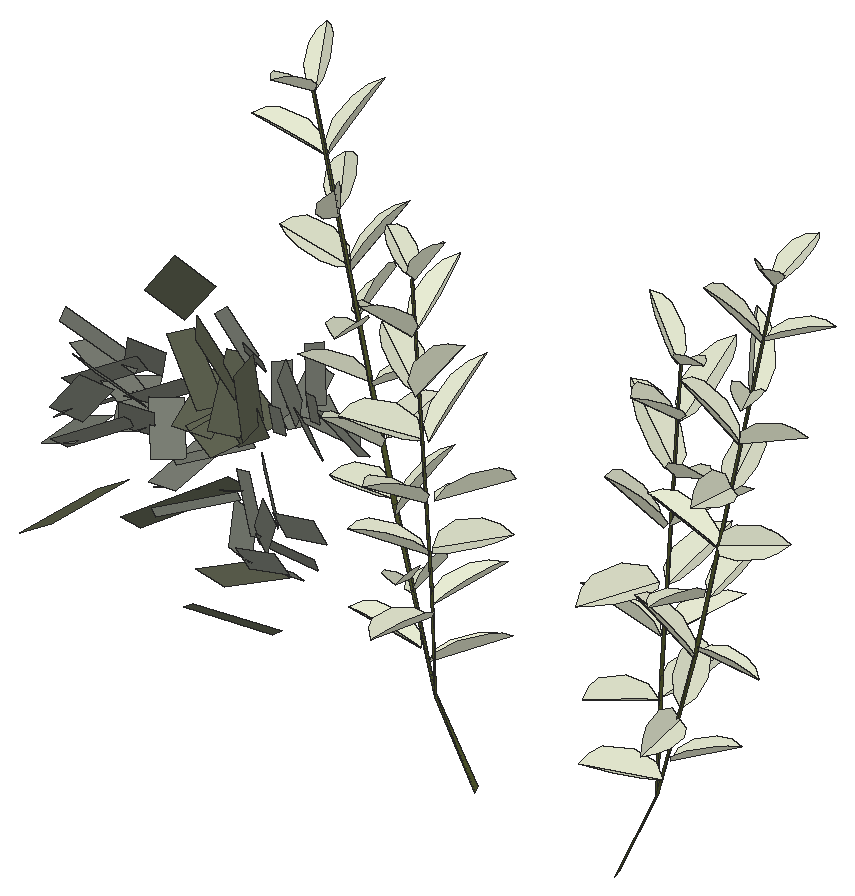
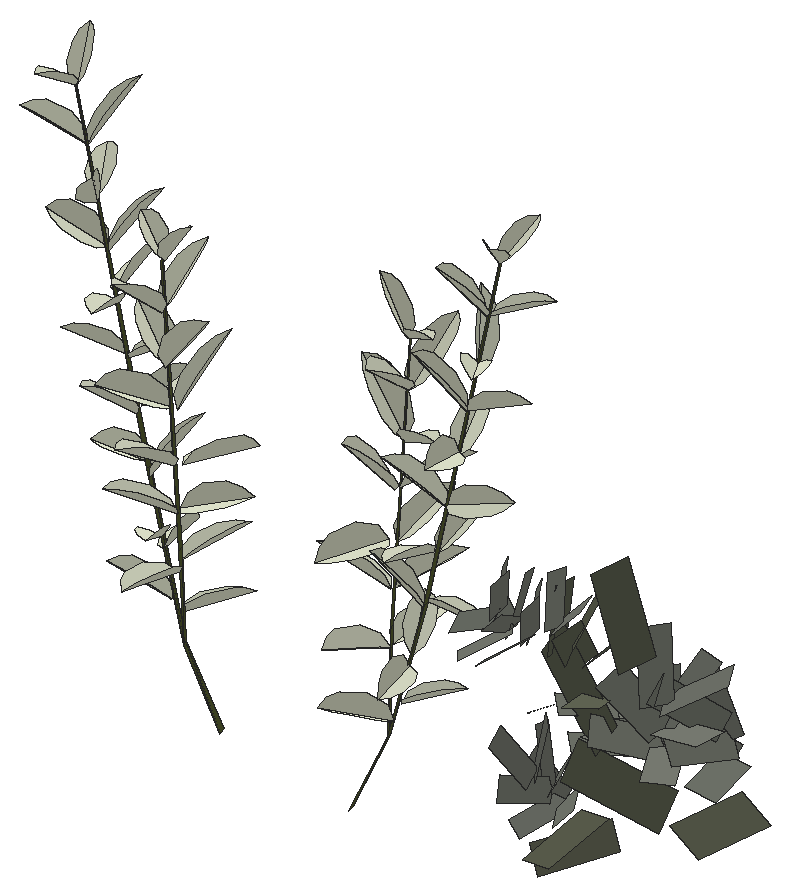
# SketchUp Ruby script. Lengths in inches.
U = 1.inch
M = Sketchup.active_model
def pt(a) = Geom::Point3d.new(a.map { |v| v * U })
def face(e, loops, mat)
  f = e.add_face(loops[0].map { |a| pt(a) })
  loops[1..].each { |l| e.add_face(l.map { |a| pt(a) }).erase! }
  f.material = f.back_material = mat if mat
  f
end
# faces: each face lists its corners as indices into pts; further lists are holes
def faces(e, pts, list, mat = nil) = list.each { |f| face(e, (f[0].is_a?(Array) ? f : [f]).map { |l| l.map { |i| pts[i] } }, mat) }
# xy, xz, yz: faces in a plane at the given z, y or x. An outline is a flat list of corners, or four numbers for a rectangle; further outlines are holes
def ring(l) = l.size == 4 ? [[l[0], l[1]], [l[2], l[1]], [l[2], l[3]], [l[0], l[3]]] : l.each_slice(2).to_a
def flat(e, list, mat, &to3) = list.each { |f| face(e, (f[0].is_a?(Array) ? f : [f]).map { |l| ring(l).map { |u, v| to3.(u, v) } }, mat) }
def xy(e, z, list, mat = nil) = flat(e, list, mat) { |x, y| [x, y, z] }
def xz(e, y, list, mat = nil) = flat(e, list, mat) { |x, z| [x, y, z] }
def yz(e, x, list, mat = nil) = flat(e, list, mat) { |y, z| [x, y, z] }
def lines(e, pts, list) = list.each { |a, b| e.add_line(pt(pts[a]), pt(pts[b])) }
# prism: a flat outline (further loops are holes) pulled along v
def prism(e, loops, v, mat = nil)
  f = face(e, loops, mat); d = Geom::Vector3d.new(v.map { |x| x * U })
  f.pushpull(f.normal.samedirection?(d) ? d.length : -d.length)
end
def box(e, o, s, mat = nil) = prism(e, [[o, [o[0] + s[0], o[1], o[2]], [o[0] + s[0], o[1] + s[1], o[2]], [o[0], o[1] + s[1], o[2]]]], [0, 0, s[2]], mat)
def at(x, y, z, deg = 0) = Geom::Transformation.translation(pt([x, y, z])) * Geom::Transformation.rotation(ORIGIN, Z_AXIS, deg.degrees)
def axes(o, x, y, z) = Geom::Transformation.new([*x, 0, *y, 0, *z, 0, *pt(o).to_a, 1])
def part(name) = M.definitions.add(name)
# library, detail: a bought-in or finely detailed component or shape, given as its bounding box
def library(name, o, s) = part(name).tap { |d| box(d.entities, o, s) }
def detail(e, o, s) = box(e.add_group.entities, o, s)
def put(e, d, t, mat = nil) = e.add_instance(d, t).tap { |i| i.material = mat if mat }
def group(e, t, mat = nil) = e.add_group.tap { |g| g.transformation = t; g.material = mat if mat }.entities
root = M.entities
M.materials.add("asdfasdf0165f6asdLeafVar1sfd015as60f1as6").color = [231, 235, 211]
M.materials.add("dw_stemssadfasdfa0sdf1s01d6w1").color = [90, 97, 50]
M.materials.add("viburnumblaasdfas0df1w06d").color = [98, 102, 84]
M.materials.add("viburnumbladsadfasdfad0w122").color = [125, 129, 119]
c1 = part("vdw_leaf\#3")
p = [[0,0,0],[-2.77,1.61,2.32],[-4.3125,6.1,4.5],[-3.97,13.49,6.09],[-2.47,18.57,6.3],[-0.2,22.73,5.75],
  [2.54,19.66,6.85],[4.3,15.93,7.09],[5.03,7.6,5.43],[3.32,1.76,2.74]]
faces(c1.entities,p,[[0,1,2,3,4,5],[0,5,6,7,8,9]],"asdfasdf0165f6asdLeafVar1sfd015as60f1as6")
c2 = part("dw_brancj_2\#2")
p = [[9.7,-0.22,29.95],[0.23,-1.96,0.34],[-0.05,1.51,0.11],[9.65,1.51,29.46],[18.64,-8.75,84.43],[18.96,-6.63,84.625],
  [1.53,6.02,63.68],[1.42,8.18,63.25],[-10.58,8.77,161.17],[-10.41,9.98,160.68],[26.34,-9.37,211.72],[26.57,-8.28,211.23]]
faces(c2.entities,p,[[0,1,2],[0,2,3],[4,0,3],[4,3,5],[6,0,3],[6,3,7],[8,6,7],[8,7,9],
  [10,4,5],[10,5,11]],"dw_stemssadfasdfa0sdf1s01d6w1")
c3 = part("vdw_branch2\#3")
put(c3.entities,c1,axes([19.53,-5.9,102.42],[1.12377,-0.50004,0],[0.46097,1.03596,0.47664],[-0.19377,-0.43548,1.13389]))
put(c3.entities,c1,axes([-5.89,6.52,109.44],[-1.07209,0.83679,0],[-0.77141,-0.98832,0.52702],[0.32427,0.41545,1.25373]))
put(c3.entities,c1,axes([-0.44,8.23,75.28],[0.88709,-0.9947,0],[0.92159,0.82189,0.33087],[-0.25219,-0.22491,1.26111]))
put(c3.entities,c1,axes([24.71,-8.97,190.81],[-0.82641,0.91101,0],[-0.83983,-0.76184,0.47664],[0.35303,0.32025,1.13389]))
put(c3.entities,c1,axes([-2.29,8.24,91.35],[1.24603,-0.47303,0],[0.43826,1.15445,0.33087],[-0.11993,-0.31592,1.26111]))
put(c3.entities,c1,axes([12.26,-3.11,37.92],[-0.64625,1.02205,0.22511],[-1.04383,-0.61044,-0.22511],[-0.07533,-0.30931,1.18809]))
put(c3.entities,c1,axes([26.17,-9.17,210.27],[-0.99452,-0.10453,0],[0.09636,-0.91681,0.38752],[-0.04051,0.38539,0.92186]))
put(c3.entities,c1,axes([-6.07,9.4,125.35],[-0.90214,-0.98107,0],[0.90896,-0.83583,0.33087],[-0.24874,0.22873,1.26111]))
put(c3.entities,c1,axes([-4.13,7.29,110.58],[0.44715,-1.078,0.64369],[1.05816,0.63649,0.33087],[-0.58725,0.40856,1.09216]))
put(c3.entities,c1,axes([23.91,-8.22,171.96],[0.62307,0.85009,-0.63406],[-0.71531,0.8798,0.47664],[0.78296,0.12729,0.94004]))
put(c3.entities,c2,at(-0.09,0.18,-0.25),"dw_stemssadfasdfa0sdf1s01d6w1")
put(c3.entities,c1,axes([23.34,-9.65,156.59],[-0.31364,-1.00782,0.58216],[1.10369,-0.17062,0.29925],[-0.17137,0.6239,0.98776]))
put(c3.entities,c1,axes([15.03,-3.37,58.83],[-1.05425,-0.00194,0.58442],[-0.14303,-1.11707,-0.26172],[0.55355,-0.3046,0.99755]))
put(c3.entities,c1,axes([-11.625,9.46,160.37],[0.36812,0.92978,0],[-0.85713,0.33936,0.38752],[0.3603,-0.14265,0.92186]))
put(c3.entities,c1,axes([21.32,-8.53,138.72],[1.21379,0.19904,0],[-0.19904,1.21379,0],[0,0,1.23]))
put(c3.entities,c1,axes([22.54,-9.2,141.43],[-1.02887,0.17955,0.60182],[-0.23387,-1.13057,-0.06253],[0.56696,-0.17376,1.02111]))
put(c3.entities,c1,axes([23.9,-8.82,173.84],[-1.14567,-0.37474,0],[0.35918,-1.0981,0.04438],[-0.01409,0.04308,1.17993]))
put(c3.entities,c1,axes([-7.84,8.92,143.59],[-1.26971,0.40522,0],[-0.37543,-1.17638,0.33087],[0.10274,0.32192,1.26111]))
put(c3.entities,c1,axes([19.77,-8.01,85.98],[-0.32405,-1.14591,0.18674],[1.10278,-0.32969,-0.10948],[0.15845,0.14442,1.16117]))
put(c3.entities,c1,axes([-0.62,5.76,76.34],[-0.08879,1.17576,-0.67771],[-1.34525,-0.16582,-0.11144],[-0.17897,0.66309,1.17383]))
put(c3.entities,c1,axes([20.49,-8.22,121.07],[0.39924,-0.78471,-0.8233],[1.08735,0.33121,0.2116],[0.09035,-0.83005,0.83495]))
put(c3.entities,c1,axes([15.15,-3.72,62.9],[1.16251,0.40128,-0.0211],[-0.39924,1.16074,0.07874],[0.0456,-0.06757,1.2273]))
put(c3.entities,c1,axes([20.72,-8.08,120.26],[-0.03693,1.2277,-0.06551],[-1.22944,-0.03698,0],[-0.00197,0.06548,1.22825]))
put(c3.entities,c1,axes([22.58,-8.36,155.57],[-0.56247,1.09386,0],[-1.00839,-0.51852,0.47664],[0.42389,0.21796,1.13389]))
put(c3.entities,c1,axes([3.97,3.13,57.96],[-1.09459,0.76041,0],[-0.72262,-1.0402,-0.1735],[-0.10109,-0.14552,1.29352]))
put(c3.entities,c1,axes([-10.8,9.06,160.75],[-0.66334,-0.72138,0],[0.66835,-0.61458,0.24329],[-0.1829,0.16818,0.92729]))
put(c3.entities,c1,axes([19.06,-9.3125,103.96],[-1.01345,0.25553,-0.60051],[-0.2265,-1.12952,-0.09839],[-0.59598,0.03076,1.01889]))
put(c3.entities,c1,axes([18.07,-6.2,81.7],[-0.56247,1.09386,0],[-1.00839,-0.51852,0.47664],[0.42389,0.21796,1.13389]))
put(c3.entities,c1,axes([12.95,-0.39,43.31],[0.13044,-1.19832,0],[1.11025,0.12085,0.29925],[-0.30382,-0.03307,1.14057]))
put(c3.entities,c1,axes([2.28,8.28,56.18],[1.32413,-0.31027,0],[0.30923,1.31968,-0.11144],[0.02542,0.1085,1.35543]))
put(c3.entities,c1,axes([-7.55,9.96,143.07],[1.34251,-0.21744,0],[0.20045,1.23761,0.52702],[-0.08426,-0.52024,1.25373]))
put(c3.entities,c1,axes([26.15,-8.25,210.66],[0.94661,-0.25364,0],[0.235,0.87703,0.24329],[-0.06431,-0.24,0.92729]))
put(c3.entities,c1,axes([-6.48,11.37,125.16],[0.64635,1.10315,0.46356],[-1.16569,0.46153,0.52702],[0.27017,-0.6478,1.16488]))
put(c3.entities,c1,axes([25.74,-8.35,191.28],[0.13044,-1.19832,0],[1.11025,0.12085,0.29925],[-0.30382,-0.03307,1.14057]))
put(c3.entities,c1,axes([-5.125,7.47,91.6],[-1.10024,0.63688,0.48318],[-0.78682,-1.00808,-0.46292],[0.14137,-0.65404,1.184]))
c4 = part("Component\#315")
p = [[0.25,0,0],[2.05,0.01,0.35],[1.81,4.2,1.66],[0,4.19,1.3125]]
faces(c4.entities,p,[[0,1,2,3]],"viburnumbladsadfasdfad0w122")
c5 = part("viburnumblad2")
put(c5.entities,c4,axes([-19.23,-4.49,-32.18],[83.35428,0,0],[0,79.38502,0],[0,0,83.35428]))
c6 = part("Component\#314")
p = [[0.14,0,0],[2.58,0.05,0.25],[2.44,5.11,2.64],[0,5.05,2.39]]
faces(c6.entities,p,[[0,1,2,3]],"viburnumblaasdfas0df1w06d")
c7 = part("viburnumblad1\#2")
put(c7.entities,c6,axes([-37.25,6.23,19.31],[75.98784,0,0],[0,65.50676,0],[0,0,75.98784]))
put(root,c3,axes([2244.85,350.01,8.3],[0.15791,0.02906,-0.03733],[-0.02958,0.1607,0],[0.02984,0.00549,0.19757]))
put(root,c5,axes([2205.54,352.5,22.32],[-0.00906,-0.00899,0.00397],[0.00943,-0.00624,0.00738],[-0.00308,0.00772,0.01046]))
put(root,c3,axes([2232.95,352.57,8.3],[-0.15667,-0.0351,-0.03733],[0.03572,-0.15945,0],[-0.0296,-0.00663,0.19757]))
put(root,c5,axes([2212.17,352.17,20.5625],[-0.00007,-0.01222,0.00309],[0.01323,-0.00017,-0.00035],[0.00036,0.00309,0.01221]))
put(root,c5,axes([2204.85,351.98,20.74],[0.00073,-0.01105,0.00534],[0.01289,0.00219,0.00278],[-0.00345,0.00543,0.01171]))
put(root,c7,axes([2204.25,348.69,15.78],[0.01294,-0.00163,0.0067],[0.00488,0.01526,-0.00571],[-0.00546,0.00626,0.01208]))
put(root,c5,axes([2209.11,354.23,21.94],[-0.01116,-0.00699,0.00046],[0.007,-0.01076,0.00634],[-0.00299,0.00562,0.01283]))
put(root,c5,axes([2209.12,353.81,23.82],[-0.01381,0.0032,-0.00202],[-0.0038,-0.01243,0.00635],[-0.00034,0.00659,0.01271]))
put(root,c5,axes([2211.26,351.42,19.3],[0.00841,-0.00866,0.00086],[0.00975,0.00926,-0.00213],[0.0008,0.00201,0.01242]))
put(root,c5,axes([2218.92,353.78,25.2],[-0.0065,0.00265,0.00695],[0.00166,-0.0098,0.00501],[0.00741,0.00415,0.00458]))
put(root,c7,axes([2216.77,352.36,24.61],[-0.00255,0.011,0.00125],[-0.00551,-0.00279,0.01135],[0.00975,0.00148,0.00412]))
put(root,c5,axes([2220.97,354.26,26.42],[-0.00677,0.00276,0.00724],[0.00154,-0.00908,0.00464],[0.00741,0.00415,0.00458]))
put(root,c5,axes([2203.77,351.0625,21],[0.0138,0.00142,0.00148],[-0.00058,0.0109,-0.00504],[-0.00186,0.00548,0.01205]))
put(root,c5,axes([2219.78,354.65,25.67],[-0.00435,-0.00477,0.00798],[0.00611,-0.00825,-0.00162],[0.00685,0.00405,0.00535]))
put(root,c7,axes([2215.27,353.36,26.25],[-0.00734,0.00868,0.00063],[-0.0075,-0.00708,0.00798],[0.0058,0.00404,0.00785]))
put(root,c5,axes([2211.48,351.05,22.65],[0.00886,0.00826,-0.00347],[-0.00846,0.00932,0.00058],[0.00295,0.00192,0.0121]))
put(root,c5,axes([2208.85,355.32,25.1875],[-0.01238,-0.00695,0.00189],[0.007,-0.01076,0.00634],[-0.00166,0.00641,0.0127]))
put(root,c5,axes([2211.1,351.33,20.97],[0.01246,-0.00054,-0.00182],[0.00031,0.0125,-0.00159],[0.00187,0.00153,0.01237]))
put(root,c5,axes([2204.46,353.55,23.51],[0.00041,-0.01136,0.00703],[0.01289,0.00219,0.00278],[-0.00352,0.00669,0.01102]))
put(root,c5,axes([2211.75,352.5625,22.23],[0.00876,-0.00902,0.0009],[0.00903,0.00857,-0.00197],[0.0008,0.00201,0.01242]))
put(root,c5,axes([2203.68,352.29,22.09],[0.00964,-0.00707,0.00598],[0.00804,0.00897,-0.00235],[-0.00301,0.00576,0.01168]))
put(root,c7,axes([2212.52,352.1875,12.66],[0.00779,-0.00697,0.00615],[0.01029,0.00367,-0.00887],[0.00279,0.00941,0.00713]))
put(root,c5,axes([2219.77,353.6,26.18],[-0.00523,0.00868,0.00226],[-0.00357,-0.00459,0.00897],[0.00802,0.00357,0.00411]))
put(root,c7,axes([2213.84,352.23,25.35],[0.00125,0.01083,-0.00332],[-0.01199,0.00283,0.0046],[0.00457,0.00236,0.00909]))
put(root,c5,axes([2208.1,353.77,25.73],[-0.00715,0.01146,-0.00475],[-0.01239,-0.00628,0.0035],[0.00072,0.00585,0.01305]))
put(root,c5,axes([2215.7,354.73,15.48],[-0.00478,-0.00491,0.00751],[0.00915,-0.00588,0.00198],[0.00339,0.00769,0.00718]))
put(root,c7,axes([2214.77,351.91,24.56],[0.00373,0.00907,-0.00579],[-0.00694,0.00792,0.00773],[0.00862,0.00055,0.00603]))
put(root,c5,axes([2216.18,355.3125,27.74],[-0.00905,-0.00157,0.00381],[0.00376,-0.00932,0.00479],[0.00255,0.00548,0.00745]))
put(root,c7,axes([2208.52,353.2,15.64],[0.00205,-0.01309,0.00844],[0.0176,0.00417,0.0022],[-0.00351,0.00791,0.01312]))
put(root,c5,axes([2216.69,354.97,16.5625],[-0.00948,0.00167,0.00544],[0.00331,-0.00711,0.00795],[0.00466,0.00836,0.00554]))
put(root,c5,axes([2208.11,355.41,23.11],[-0.0037,-0.01302,0.00469],[0.0125,-0.00235,0.00334],[-0.00247,0.0054,0.01303]))
put(root,c5,axes([2218.34,353.28,26.26],[-0.00065,0.00993,-0.00423],[-0.00522,0.0028,0.00703],[0.00831,0.00266,0.0042]))
put(root,c5,axes([2220.41,355.45,26.53],[0.00062,-0.00952,0.00405],[0.00764,-0.00238,-0.00656],[0.00666,0.00333,0.00596]))
put(root,c7,axes([2211.4,355.36,20.78],[-0.01053,-0.00014,0.0139],[0.01206,-0.01352,0.00899],[0.00923,0.01297,0.00712]))
put(root,c5,axes([2207.41,353.15,23.98],[0.0037,0.01302,-0.00469],[-0.01381,0.00379,-0.00038],[0.0009,0.00462,0.01353]))
put(root,c7,axes([2212.19,352.14,23.66],[0.01142,0.00359,-0.00296],[-0.00486,0.01317,-0.00274],[0.00185,0.00298,0.01066]))
put(root,c7,axes([2212.63,352.47,23.64],[0.00961,-0.00181,-0.00747],[-0.00022,0.01383,-0.00363],[0.00726,0.00235,0.00826]))
put(root,c5,axes([2215.53,354.41,28.44],[-0.00329,0.00963,-0.00365],[-0.0081,-0.00098,0.00442],[0.00408,0.00455,0.00739]))
put(root,c5,axes([2220.3125,353.86,27.47],[-0.00062,0.00952,-0.00405],[-0.0058,0.00311,0.00781],[0.00831,0.00266,0.0042]))
put(root,c5,axes([2207.69,354.71,21.5625],[0.00747,-0.01197,0.00496],[0.01097,0.00676,-0.00022],[-0.0023,0.00416,0.01351]))
put(root,c7,axes([2208.75,356.49,27.58],[-0.01185,-0.00554,0.00715],[0.01005,-0.01197,0.00738],[0.00259,0.00922,0.01142]))
put(root,c7,axes([2213.09,352.87,14.73],[0.01169,-0.00232,-0.00224],[0.00035,0.01065,-0.00919],[0.00321,0.00758,0.00891]))
put(root,c5,axes([2216.91,356.44,17.11],[-0.0048,-0.00448,0.0089],[0.00915,-0.00588,0.00198],[0.00393,0.00822,0.00626]))
put(root,c5,axes([2214.62,354.96,15.92],[0.00898,-0.00714,0.00125],[0.00484,0.00482,-0.00724],[0.0044,0.00684,0.00749]))
put(root,c5,axes([2218.91,355.18,26.51],[0.00523,-0.00868,-0.00226],[0.00529,0.00516,-0.00737],[0.00696,0.00241,0.00605]))
put(root,c5,axes([2215.47,355.91,16.375],[0.00269,-0.008,0.00714],[0.0092,-0.00069,-0.00424],[0.00383,0.00759,0.00707]))
put(root,c5,axes([2218.97,353.83,27.07],[0.00435,0.00477,-0.00798],[-0.00392,0.00825,0.00263],[0.00812,0.00193,0.0048]))
put(root,c5,axes([2217.04,355.48,18.11],[-0.0086,0.00684,-0.0012],[-0.00415,-0.00354,0.00962],[0.00557,0.00793,0.00532]))
put(root,c5,axes([2215.92,354.53,17.67],[-0.00269,0.008,-0.00714],[-0.00879,0.00257,0.00619],[0.00614,0.00718,0.00574]))
put(root,c5,axes([2207.08,353.07,22.09],[0.01189,0.00667,-0.00181],[-0.00777,0.01295,-0.00333],[0.00008,0.00361,0.01386]))
put(root,c5,axes([2217.89,354.29,26.43],[0.00544,-0.00271,-0.00718],[0.0003,0.00981,-0.00339],[0.00825,0.00152,0.00476]))
put(root,c5,axes([2214.84,353.9375,16.86],[0.00461,0.0043,-0.00854],[-0.00856,0.00831,-0.00043],[0.00603,0.00655,0.00655]))
